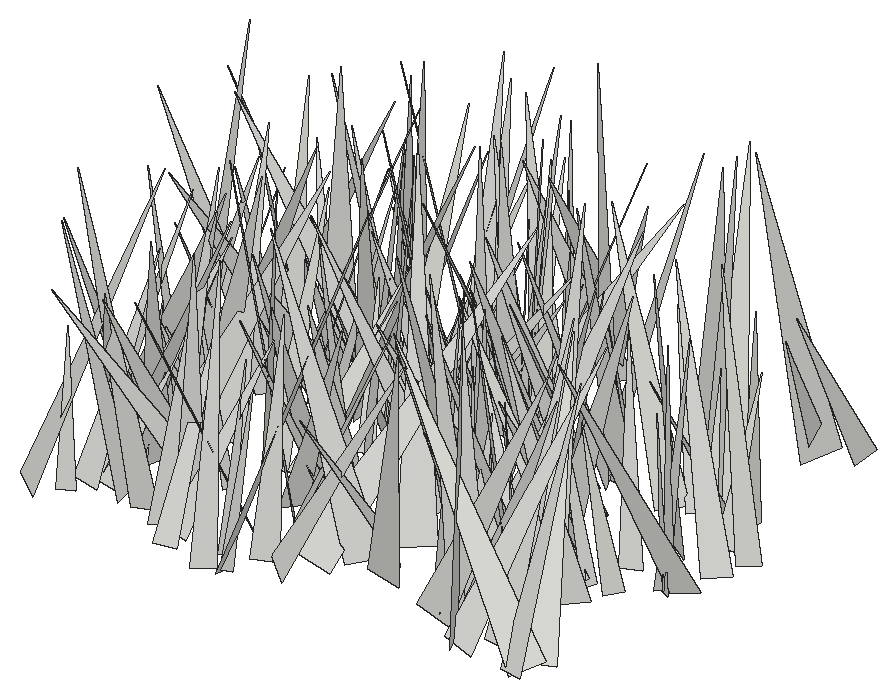
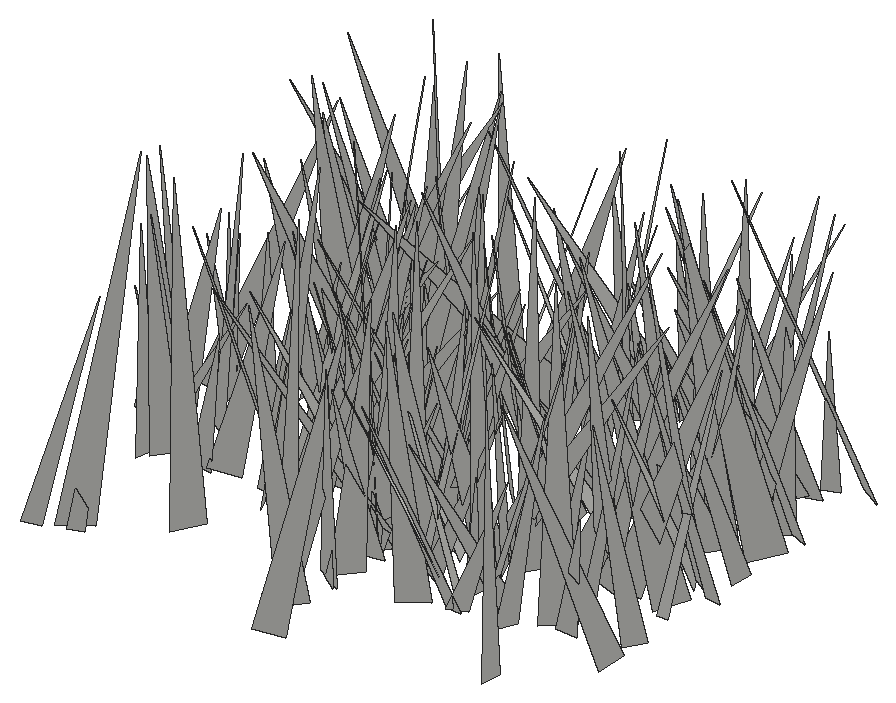
# SketchUp Ruby script. Lengths in inches.
U = 1.inch
M = Sketchup.active_model
def pt(a) = Geom::Point3d.new(a.map { |v| v * U })
def face(e, loops, mat)
  f = e.add_face(loops[0].map { |a| pt(a) })
  loops[1..].each { |l| e.add_face(l.map { |a| pt(a) }).erase! }
  f.material = f.back_material = mat if mat
  f
end
# faces: each face lists its corners as indices into pts; further lists are holes
def faces(e, pts, list, mat = nil) = list.each { |f| face(e, (f[0].is_a?(Array) ? f : [f]).map { |l| l.map { |i| pts[i] } }, mat) }
# xy, xz, yz: faces in a plane at the given z, y or x. An outline is a flat list of corners, or four numbers for a rectangle; further outlines are holes
def ring(l) = l.size == 4 ? [[l[0], l[1]], [l[2], l[1]], [l[2], l[3]], [l[0], l[3]]] : l.each_slice(2).to_a
def flat(e, list, mat, &to3) = list.each { |f| face(e, (f[0].is_a?(Array) ? f : [f]).map { |l| ring(l).map { |u, v| to3.(u, v) } }, mat) }
def xy(e, z, list, mat = nil) = flat(e, list, mat) { |x, y| [x, y, z] }
def xz(e, y, list, mat = nil) = flat(e, list, mat) { |x, z| [x, y, z] }
def yz(e, x, list, mat = nil) = flat(e, list, mat) { |y, z| [x, y, z] }
def lines(e, pts, list) = list.each { |a, b| e.add_line(pt(pts[a]), pt(pts[b])) }
# prism: a flat outline (further loops are holes) pulled along v
def prism(e, loops, v, mat = nil)
  f = face(e, loops, mat); d = Geom::Vector3d.new(v.map { |x| x * U })
  f.pushpull(f.normal.samedirection?(d) ? d.length : -d.length)
end
def box(e, o, s, mat = nil) = prism(e, [[o, [o[0] + s[0], o[1], o[2]], [o[0] + s[0], o[1] + s[1], o[2]], [o[0], o[1] + s[1], o[2]]]], [0, 0, s[2]], mat)
def at(x, y, z, deg = 0) = Geom::Transformation.translation(pt([x, y, z])) * Geom::Transformation.rotation(ORIGIN, Z_AXIS, deg.degrees)
def axes(o, x, y, z) = Geom::Transformation.new([*x, 0, *y, 0, *z, 0, *pt(o).to_a, 1])
def part(name) = M.definitions.add(name)
# library, detail: a bought-in or finely detailed component or shape, given as its bounding box
def library(name, o, s) = part(name).tap { |d| box(d.entities, o, s) }
def detail(e, o, s) = box(e.add_group.entities, o, s)
def put(e, d, t, mat = nil) = e.add_instance(d, t).tap { |i| i.material = mat if mat }
def group(e, t, mat = nil) = e.add_group.tap { |g| g.transformation = t; g.material = mat if mat }.entities
root = M.entities
c1 = part("fur_instance\#9")
p = [[0.8125,0,1.79],[0.67,-0.02,1.48],[0,-0.11,0],[0,0.11,0]]
faces(c1.entities,p,[[0,1,2,3]])
put(root,c1,axes([86.75,304.64,-27.1],[-1.48065,3.15767,1.46809],[3.42197,1.61497,-0.02236],[0.64523,-1.31889,3.48751]))
put(root,c1,axes([94.63,306.8,-27.1],[-3.64802,-5.0358,0.07825],[-5.03596,3.64854,0.02575],[0.06676,0.04827,6.21825]))
put(root,c1,axes([101.23,306.93,-27.1],[0.69431,-7.1025,1.01226],[-6.95299,-0.41552,1.85354],[1.7681,1.15502,6.89145]))
put(root,c1,axes([110.4,304.75,-27.1],[-5.51381,4.9525,0.02994],[4.6746,5.18943,2.47955],[-1.63592,-1.86355,6.98435]))
put(root,c1,axes([91.37,308.08,-27.1],[-6.30471,-1.37126,0.42808],[-1.05468,5.72683,2.8114],[0.97532,-2.67133,5.80738]))
put(root,c1,axes([88.87,305.9375,-27.1],[-6.26748,-0.84521,1.62615],[-0.68504,6.45447,0.7145],[1.69984,-0.51518,6.28372]))
put(root,c1,axes([106.66,304.7,-27.1],[6.19858,3.66698,3.16063],[3.75526,-6.8827,0.6206],[-3.05522,-1.01998,7.17523]))
put(root,c1,axes([95.93,303.48,-27.1],[-3.80527,0.70423,0.62745],[0.3357,3.44844,-1.83447],[0.88144,1.72686,3.40746]))
put(root,c1,axes([97.41,304.875,-27.1],[3.70489,5.29932,0.63458],[5.07029,-3.25343,-2.43293],[1.66665,-1.88258,5.99082]))
put(root,c1,axes([95.1,303.0625,-27.1],[-5.93651,2.05948,0.4431],[1.83167,5.70073,-1.95618],[1.04056,1.71471,5.97135]))
put(root,c1,axes([96.62,305.09,-27.1],[-2.20726,4.7722,2.01563],[5.04733,2.47451,-0.33147],[1.16667,-1.67676,5.24748]))
put(root,c1,axes([100.51,308.8,-27.1],[-3.99829,-3.957,0.07334],[-3.50173,3.58563,2.55553],[1.84422,-1.77059,5.01133]))
put(root,c1,axes([90.21,305.41,-27.1],[-1.59145,-6.67923,2.98055],[-7.18236,0.85085,-1.92829],[-1.38185,3.26993,6.58988]))
put(root,c1,axes([85.25,304,-27.1],[4.54632,6.46757,0.61256],[6.48609,-4.47646,-0.87508],[0.36794,-1.0028,7.85702]))
put(root,c1,axes([104.68,305.83,-27.1],[2.05152,-6.6713,2.37008],[-6.64568,-0.96384,3.03943],[2.44098,2.98279,6.28306]))
put(root,c1,axes([95.06,304.51,-27.1],[-3.85021,0.78609,0.9669],[0.45373,3.80886,-1.28983],[1.16059,1.11875,3.71193]))
put(root,c1,axes([92.46,304.58,-27.1],[0.05703,4.78722,0.58826],[4.57544,0.13244,-1.52137],[1.52606,-0.57598,4.5394]))
put(root,c1,axes([91.9375,306.15,-27.1],[5.0258,-2.8928,2.35137],[-3.11716,-5.42578,-0.01254],[-2.04464,1.16127,5.79886]))
put(root,c1,axes([92.71,303.54,-27.1],[-4.05374,2.9207,0.15477],[2.65047,3.78022,-1.91631],[1.23673,1.47198,4.61422]))
put(root,c1,axes([108.58,306.6875,-27.1],[-4.58076,1.47717,0.18742],[1.47131,4.39705,1.30451],[-0.22897,-1.29786,4.63288]))
put(root,c1,axes([110.08,304.04,-27.1],[1.80185,5.93958,0.37976],[5.89361,-1.83593,0.75111],[-0.82954,-0.14229,6.16126]))
put(root,c1,axes([89.45,309.17,-27.1],[5.03177,-2.92165,1.14225],[-2.20313,-4.82824,-2.64459],[-2.23316,-1.81978,5.18275]))
put(root,c1,axes([86.01,308.63,-27.1],[5.48383,-1.63022,0.30334],[-1.45467,-5.23263,-1.82362],[-0.79597,-1.66854,5.42259]))
put(root,c1,axes([88.15,308.71,-27.1],[6.15158,-3.29467,0.71793],[-3.15743,-6.15236,-1.17953],[-1.18361,-0.7112,6.87789]))
put(root,c1,axes([87,305.6,-27.1],[0.12132,5.40428,1.16344],[5.42728,0.10479,-1.05269],[1.05091,-1.16504,5.30215]))
put(root,c1,axes([105.55,306.79,-27.1],[-7.11208,1.53537,2.26223],[1.65379,7.4363,0.15223],[2.17716,-0.6331,7.27433]))
put(root,c1,axes([105.69,307.03,-27.1],[3.10657,-5.20372,2.6425],[-5.63717,-3.45056,-0.16782],[-1.51121,2.17421,6.05816]))
put(root,c1,axes([107.08,304.44,-27.1],[1.06363,7.1406,0.14161],[6.98782,-1.01087,-1.51263],[1.47601,-0.35985,7.05914]))
put(root,c1,axes([105.9,306.92,-27.1],[5.04993,-3.13211,0.88061],[-3.25342,-4.87587,1.31476],[-0.02926,1.58216,5.79512]))
put(root,c1,axes([95.79,303.2,-27.1],[6.81061,4.1437,0.72104],[3.52808,-6.3754,3.31382],[-2.28972,2.50169,7.25074]))
put(root,c1,axes([91.59,304.95,-27.1],[-6.63675,3.07759,1.929],[2.57186,6.8191,-2.03087],[2.56478,1.12578,7.02806]))
put(root,c1,axes([108.1,306.99,-27.1],[-5.99226,-3.56649,1.99916],[-3.93709,5.99,-1.11487],[1.10264,2.00593,6.88361]))
put(root,c1,axes([99.76,307.56,-27.1],[-4.16416,5.80884,2.0419],[6.1268,3.66414,2.07088],[-0.6118,-2.84317,6.84063]))
put(root,c1,axes([103.8,310.01,-27.1],[-0.44109,-6.89492,0.21564],[-6.89758,0.44393,0.08524],[0.09888,0.20974,6.90849]))
put(root,c1,axes([87.5,306.84,-27.1],[6.84085,-1.05323,0.60817],[-1.14548,-6.7472,1.19982],[-0.40871,1.28156,6.81667]))
put(root,c1,axes([108.29,305.54,-27.1],[1.00933,7.00307,0.82634],[7.04916,-1.02422,0.06983],[-0.18746,-0.80782,7.07509]))
put(root,c1,axes([87.49,306.01,-27.1],[-0.99691,5.86129,1.26655],[5.41282,1.43213,-2.36709],[2.58075,-0.73958,5.45394]))
put(root,c1,axes([105.18,307.28,-27.1],[2.53545,-3.02814,1.98338],[-3.53036,-2.60371,0.53779],[-0.80002,1.89288,3.91266]))
put(root,c1,axes([108.45,308.1,-27.1],[-2.5015,-6.23633,1.72664],[-6.18785,1.76379,-2.59425],[-1.89304,2.47545,6.19832]))
put(root,c1,axes([110.48,305.32,-27.1],[-3.69849,5.78351,0.10997],[5.76561,3.69627,-0.48502],[0.46777,0.16892,6.84781]))
put(root,c1,axes([87.125,309.52,-27.1],[-0.56263,-5.96411,0.83016],[-5.9756,0.45013,-0.816],[-0.74291,0.89616,5.93475]))
put(root,c1,axes([95.91,307.79,-27.1],[5.05169,2.87341,0.23488],[2.86098,-4.93803,-1.1233],[0.35552,-1.09113,5.70213]))
put(root,c1,axes([95.61,310.51,-27.1],[-4.40501,-3.46188,0.56585],[-3.18391,4.32713,1.68747],[1.47225,-1.00011,5.34239]))
put(root,c1,axes([104.59,306.125,-27.1],[3.23969,5.31398,1.47982],[4.81259,-3.56155,2.25346],[-2.69577,0.02794,5.80137]))
put(root,c1,axes([95.23,308.68,-27.1],[-5.96506,-5.04673,2.13711],[-5.35643,6.03696,-0.69462],[1.15994,1.92465,7.7826]))
put(root,c1,axes([87.87,308.01,-27.1],[1.06055,3.50039,1.15885],[3.68372,-1.05849,-0.17402],[-0.16095,-1.16074,3.65339]))
put(root,c1,axes([106.7,308.75,-27.1],[-3.07228,-3.20464,1.70758],[-3.41257,3.31254,0.07678],[1.24093,1.17551,4.43878]))
put(root,c1,axes([94.75,309.3,-27.1],[4.6953,-3.04636,0.27903],[-3.0591,-4.67738,0.40996],[-0.01004,0.49581,5.58194]))
put(root,c1,axes([103.18,309.26,-27.1],[-1.62958,-3.15436,1.09529],[-3.33909,1.53504,-0.54711],[-0.01197,1.22427,3.50802]))
put(root,c1,axes([92.86,309.88,-27.1],[6.58164,2.52237,2.667],[2.99732,-6.85363,-0.91486],[-2.11926,-1.85972,6.9888]))
put(root,c1,axes([108.49,310.15,-27.1],[-3.08305,4.83073,2.80211],[5.58378,2.72141,1.452],[0.09585,-3.15451,5.54372]))
put(root,c1,axes([107.08,308.8,-27.1],[-4.22119,3.06488,0.48562],[3.10212,4.18863,0.52921],[0.07866,-0.71394,5.1896]))
put(root,c1,axes([85.35,310.52,-27.1],[4.73655,-6.32836,0.37656],[-6.13582,-4.45802,2.25891],[1.59428,1.644,7.57499]))
put(root,c1,axes([87.41,310.73,-27.1],[0.83878,-6.84447,1.51714],[-6.71971,-0.34936,2.13903],[1.99848,1.69801,6.55552]))
put(root,c1,axes([85.33,308.53,-27.1],[3.14685,5.37097,0.90824],[5.43729,-3.03382,-0.89816],[0.32882,-1.23429,6.15981]))
put(root,c1,axes([88.83,311.11,-27.1],[2.63547,-2.52355,0.88422],[-2.24578,-2.7628,-1.19134],[-1.45143,-0.30736,3.44888]))
put(root,c1,axes([94.06,311.8,-27.1],[0.0355,-6.28923,0.69696],[-6.32457,-0.05728,-0.19472],[-0.19984,0.69551,6.28631]))
put(root,c1,axes([89.85,308.79,-27.1],[-6.30755,-1.0303,0.95825],[-1.23667,6.15876,-1.51833],[0.67114,1.66527,6.20817]))
put(root,c1,axes([91.82,308.8,-27.1],[-4.16837,-0.36819,0.02902],[-0.35612,3.91965,-1.4217],[-0.09791,1.41863,3.93569]))
put(root,c1,axes([101.26,312.25,-27.1],[-1.0754,-7.3325,1.08617],[-7.40599,1.10888,0.15329],[0.31086,1.05196,7.40935]))
put(root,c1,axes([95.22,312.34,-27.1],[3.85472,-3.45884,0.89823],[-3.26491,-3.94586,-1.18314],[-1.45282,-0.30973,5.04209]))
put(root,c1,axes([98.12,306.18,-27.1],[-4.06981,7.2471,0.38585],[5.9474,3.58401,-4.58433],[4.15906,1.9665,6.9331]))
put(root,c1,axes([111.46,313.57,-27.1],[1.05272,-6.58483,0.46236],[-6.33643,-1.13928,-1.79827],[-1.85027,0.15508,6.42141]))
put(root,c1,axes([109.25,311.74,-27.1],[2.35364,-2.97334,1.61897],[-3.0072,-2.74184,-0.66374],[-1.55518,0.80187,3.73361]))
put(root,c1,axes([105.82,313.24,-27.1],[1.37303,-5.10418,0.31363],[-5.09334,-1.39399,-0.38851],[-0.45708,0.20095,5.27134]))
put(root,c1,axes([102.78,310.7,-27.1],[1.15906,3.62365,1.13013],[3.60388,-1.42153,0.86183],[-1.19166,-0.77453,3.7056]))
put(root,c1,axes([106.47,310.68,-27.1],[5.95771,-4.00613,4.25574],[-5.13988,-6.48421,1.09155],[-2.78246,3.40011,7.09591]))
put(root,c1,axes([87.35,313.3125,-27.1],[2.07111,-6.85146,1.31632],[-6.80663,-1.68294,1.94991],[1.53132,1.78604,6.88693]))
put(root,c1,axes([108.1,311.6,-27.1],[-4.0966,0.35691,0.30901],[0.31396,4.07547,-0.54495],[0.35257,0.51784,4.07585]))
put(root,c1,axes([103.57,313.69,-27.1],[-0.91918,-4.72146,0.08029],[-4.18667,0.777,-2.23865],[-2.18412,0.49761,4.25741]))
put(root,c1,axes([96.03,311.35,-27.1],[-5.27526,-0.92635,0.94955],[-1.13263,5.17215,-1.24665],[0.69057,1.40673,5.20887]))
put(root,c1,axes([104.77,314.49,-27.1],[2.5877,-3.76016,0.15432],[-3.53923,-2.49522,-1.45139],[-1.27925,-0.70276,4.32764]))
put(root,c1,axes([100.7,309.81,-27.1],[-7.32021,3.8589,0.48336],[3.73123,7.2592,-1.44642],[1.09666,1.05977,8.14767]))
put(root,c1,axes([107.57,311.35,-27.1],[-2.18408,5.95276,0.46734],[5.01759,1.55993,3.57972],[-3.2369,-1.59851,5.23366]))
put(root,c1,axes([87.36,311.43,-27.1],[0.42432,7.03314,2.02201],[6.63788,0.48281,-3.07232],[3.08094,-2.00885,6.34082]))
put(root,c1,axes([85,312.58,-27.1],[4.99939,-0.31235,0.02616],[-0.31267,-4.999,0.06629],[-0.02197,0.06779,5.0087]))
put(root,c1,axes([92.18,311.3,-27.1],[0.04484,6.03011,0.93276],[6.10111,-0.02998,-0.09948],[0.09373,-0.93336,6.02946]))
put(root,c1,axes([99.77,313.04,-27.1],[-2.20634,6.02099,1.75888],[5.48729,0.94934,3.63349],[-3.03901,-2.65713,5.28374]))
put(root,c1,axes([98.72,315.29,-27.1],[3.46257,-3.0651,1.27719],[-2.41097,-3.5895,-2.07802],[-2.28326,-0.85797,4.13111]))
put(root,c1,axes([89.42,311.83,-27.1],[-0.62472,6.74476,1.37593],[6.88336,0.62526,0.06028],[0.06565,-1.37569,6.77336]))
put(root,c1,axes([93.52,311.24,-27.1],[-0.37436,5.47936,0.25355],[5.20879,0.43477,-1.70506],[1.71934,-0.12411,5.22075]))
put(root,c1,axes([110.82,313.04,-27.1],[1.66971,3.21733,1.57549],[3.35444,-2.01427,0.55833],[-1.25742,-1.10127,3.58153]))
put(root,c1,axes([98.45,312.81,-27.1],[1.87849,6.8023,2.53671],[7.02619,-2.36292,1.13321],[-1.82724,-2.09291,6.96533]))
put(root,c1,axes([102.99,313.41,-27.1],[-3.64875,-2.02244,1.121],[-2.25149,3.58457,-0.86132],[0.52696,1.3118,4.08188]))
put(root,c1,axes([89.71,317.73,-27.1],[4.2838,-6.03866,0.74714],[-5.20831,-4.11147,-3.36808],[-3.14598,-1.41597,6.59337]))
put(root,c1,axes([98.96,313.27,-27.1],[-4.99068,-1.45127,1.21381],[-1.71677,4.91279,-1.18474],[0.79513,1.49823,5.06058]))
put(root,c1,axes([99.82,315.05,-27.1],[-0.19463,-4.95849,1.24268],[-5.00803,0.4343,0.94858],[1.02496,1.18047,4.8708]))
put(root,c1,axes([96.39,313.1,-27.1],[4.10758,4.73433,2.04961],[4.7509,-4.49256,0.85604],[-2.01089,-0.9434,6.20913]))
put(root,c1,axes([102.83,314.64,-27.1],[6.50661,-0.43072,0.76621],[-0.39332,-6.54513,-0.33931],[-0.78607,-0.29036,6.51202]))
put(root,c1,axes([104.26,317.13,-27.1],[-2.87377,-5.9267,0.11201],[-5.79461,2.83495,1.33509],[1.24935,-0.48389,6.44995]))
put(root,c1,axes([103.26,312.14,-27.1],[-3.36255,6.42423,2.20976],[5.77924,4.00105,-2.8377],[3.57129,-0.42595,6.67271]))
put(root,c1,axes([104.48,314.44,-27.1],[4.99795,-3.82327,1.26682],[-4.01963,-4.86241,1.18375],[-0.25457,1.71502,6.18026]))
put(root,c1,axes([110.68,313.48,-27.1],[-4.80095,-0.85986,1.55653],[-1.24807,4.82151,-1.18603],[1.26668,1.49164,4.73094]))
put(root,c1,axes([102.17,316.67,-27.1],[1.78326,-6.33726,0.7797],[-6.26284,-1.89367,-1.06754],[-1.24322,0.44943,6.49625]))
put(root,c1,axes([85.58,316.96,-27.1],[-2.3415,-4.6423,0.1365],[-4.37976,2.25803,1.66471],[1.54509,-0.63449,4.92568]))
put(root,c1,axes([108.52,313.74,-27.1],[-0.93822,4.8343,1.08723],[4.93478,0.81164,0.64956],[-0.44769,-1.18472,4.88147]))
put(root,c1,axes([97.93,315.9,-27.1],[4.25123,5.18566,4.75994],[6.35301,-5.22113,0.01405],[-3.03108,-3.67013,6.70551]))
put(root,c1,axes([93.1,313.26,-27.1],[8.11647,0.24258,0.67526],[0.10402,-7.98511,1.61836],[-0.70993,1.60345,7.95719]))
put(root,c1,axes([84.85,314.61,-27.1],[2.54446,5.11145,1.43196],[5.2695,-2.24073,-1.36501],[0.64019,-1.87187,5.54418]))
put(root,c1,axes([110.55,313.16,-27.1],[-4.99347,0.21503,1.45697],[-0.36457,4.80955,-1.95935],[1.42691,1.98134,4.59803]))
put(root,c1,axes([99.07,315.56,-27.1],[-2.91756,2.69263,1.56889],[3.08399,2.80363,0.92331],[0.448,-1.76443,3.86133]))
put(root,c1,axes([88.27,316.11,-27.1],[1.0703,-6.74535,2.51722],[-6.58595,-1.94546,-2.41292],[-2.90886,1.9228,6.3893]))
put(root,c1,axes([102.05,316.36,-27.1],[-4.72142,-2.258,0.83052],[-2.14472,4.77905,0.80066],[1.09019,-0.37724,5.17198]))
put(root,c1,axes([94.5,314.21,-27.1],[4.33311,5.30156,2.10924],[5.44411,-4.63436,0.46433],[-1.70794,-1.32191,6.83131]))
put(root,c1,axes([85.88,315.95,-27.1],[6.5822,-3.48627,0.04021],[-3.46978,-6.5418,0.80411],[0.34104,0.72931,7.40492]))
put(root,c1,axes([92.13,317.36,-27.1],[7.49694,-1.26912,1.50095],[-0.87324,-7.45265,-1.93987],[-1.76095,-1.70734,7.35199]))
put(root,c1,axes([104.23,314.63,-27.1],[4.8135,2.02359,1.54657],[1.94555,-5.05552,0.55956],[-1.64367,-0.05793,5.19149]))
put(root,c1,axes([98.9,315.92,-27.1],[-0.48959,-3.44443,1.08487],[-3.54488,0.6673,0.51889],[0.68909,0.98557,3.44014]))
put(root,c1,axes([103.34,316.3,-27.1],[-4.54236,-5.48641,0.31776],[-5.31376,4.27953,-2.06985],[-1.40202,1.55551,6.81539]))
put(root,c1,axes([86.07,313.93,-27.1],[3.67219,7.15908,2.03524],[7.27938,-3.92759,0.68132],[-1.55086,-1.48365,8.01705]))
put(root,c1,axes([94.33,314.5,-27.1],[-1.12302,3.48075,0.37457],[3.50037,1.10997,0.18007],[-0.0574,-0.41163,3.65299]))
put(root,c1,axes([86.4,313.78,-27.1],[4.4489,2.71988,0.66857],[2.4928,-4.41728,1.38241],[-1.27698,0.85286,5.02786]))
put(root,c1,axes([88.92,316.45,-27.1],[-1.01611,-5.1437,1.43202],[-5.3112,0.8243,-0.80778],[-0.54728,1.55038,5.1805]))
put(root,c1,axes([102.97,317.59,-27.1],[2.20766,-6.15742,1.48059],[-5.96151,-2.54967,-1.71445],[-2.13691,0.75174,6.31254]))
put(root,c1,axes([109.11,316.06,-27.1],[3.12486,4.78234,3.10342],[5.39282,-3.6275,0.15986],[-1.8492,-2.49745,5.71052]))
put(root,c1,axes([92.16,314.48,-27.1],[3.27247,4.57721,0.86039],[4.6176,-3.3258,0.13012],[-0.60735,-0.62316,5.62521]))
put(root,c1,axes([93.54,317.72,-27.1],[-7.87957,1.88276,1.17896],[2.17634,7.41366,2.70618],[0.44527,-2.91806,7.63603]))
put(root,c1,axes([96.59,317.16,-27.1],[-4.94323,1.53486,1.76986],[2.06825,4.80019,1.61379],[1.10026,-2.12747,4.91803]))
put(root,c1,axes([98.81,317.42,-27.1],[-3.02452,-1.82217,1.01563],[-1.34667,3.07159,1.50047],[1.5932,-0.86291,3.19635]))
put(root,c1,axes([96.05,315.39,-27.1],[4.06376,5.39951,0.02576],[4.83357,-3.62337,-3.0294],[2.40665,-1.8401,6.04083]))
put(root,c1,axes([95.84,318.23,-27.1],[4.75134,-2.11282,0.36953],[-1.90852,-4.57438,-1.61505],[-0.97883,-1.33672,4.94275]))
put(root,c1,axes([102.36,316.24,-27.1],[0.25275,3.74041,1.98428],[3.79537,-1.08135,1.55493],[-1.87703,-1.68284,3.41127]))
put(root,c1,axes([101.22,315.96,-27.1],[5.9616,4.7587,3.0284],[5.08757,-6.43918,0.10304],[-2.43578,-1.80245,7.62727]))
put(root,c1,axes([94.24,316.02,-27.1],[-5.6206,-6.05261,0.8091],[-5.56666,4.62654,-4.06048],[-2.5102,3.29256,7.1929]))
put(root,c1,axes([111.67,315.34,-27.1],[-1.94953,6.2532,0.70862],[6.08536,1.68405,1.8809],[-1.60411,-1.2111,6.27419]))
put(root,c1,axes([98.69,316.38,-27.1],[1.00735,6.64791,2.58508],[7.07427,-1.26504,0.49655],[-0.91221,-2.46923,6.70544]))
put(root,c1,axes([88.56,318,-27.1],[-3.05463,-4.97038,1.37571],[-5.09206,3.16016,0.11108],[0.81742,1.11209,5.83293]))
put(root,c1,axes([96.85,317.41,-27.1],[3.67258,4.04026,0.63824],[3.75616,-2.99162,-2.6759],[1.61937,-2.22383,4.75932]))
put(root,c1,axes([90,313.87,-27.1],[6.02604,4.35688,0.13616],[4.14402,-5.7981,2.12678],[-1.35204,1.64734,7.12547]))
put(root,c1,axes([103.22,318.99,-27.1],[-5.52274,-3.05851,1.02558],[-2.84433,5.57616,1.31266],[1.52186,-0.67738,6.17511]))
put(root,c1,axes([88.98,316.01,-27.1],[-0.28002,6.79198,1.74012],[7.00527,0.19856,0.35229],[-0.29175,-1.75129,6.78861]))
put(root,c1,axes([99.74,317.09,-27.1],[4.36053,2.62617,0.62372],[2.69593,-4.29581,-0.7602],[-0.13318,-0.97427,5.03319]))
put(root,c1,axes([89.6,316.79,-27.1],[5.1332,2.66859,0.80867],[2.72409,-5.16107,-0.26035],[-0.59552,-0.60587,5.77956]))
put(root,c1,axes([89.5,318.89,-27.1],[2.09335,-3.21544,0.11512],[-3.16402,-2.08217,-0.6229],[-0.58423,-0.24481,3.78592]))
put(root,c1,axes([104.1,318.88,-27.1],[-0.46017,-7.01963,1.64197],[-7.20868,0.46604,-0.02793],[0.07879,1.64032,7.03464]))
put(root,c1,axes([110.33,318.51,-27.1],[-1.30366,-3.70433,0.26528],[-3.50778,1.13584,-1.37745],[-1.21983,0.69265,3.67753]))
put(root,c1,axes([110.42,317.39,-27.1],[-0.72601,3.76819,0.7458],[3.80081,0.81458,-0.41575],[0.55615,-0.64789,3.8149]))
put(root,c1,axes([112.07,316.92,-27.1],[-0.60049,6.11637,0.8715],[5.86899,0.29123,2.00004],[-1.92986,-1.0175,5.81123]))
put(root,c1,axes([94.93,318.08,-27.1],[4.2362,2.18763,0.04516],[2.18011,-4.21144,-0.49393],[0.18673,-0.4595,4.74206]))
put(root,c1,axes([93.05,317.6,-27.1],[-5.05417,-1.27819,2.14403],[-1.86511,5.15169,-1.32541],[1.65892,1.89778,5.04199]))
put(root,c1,axes([97.76,319.55,-27.1],[6.10585,-2.9623,2.45846],[-2.96929,-6.55789,-0.52733],[-2.45002,0.56525,6.76598]))
put(root,c1,axes([106.72,318.6875,-27.1],[-3.37701,5.49526,1.43426],[5.6473,3.0721,1.52623],[-0.60248,-2.00587,6.26679]))
put(root,c1,axes([85.02,319.4,-27.1],[3.32524,-3.2763,0.88677],[-3.39381,-3.22791,0.80025],[-0.05063,1.1934,4.59902]))
put(root,c1,axes([98.41,319.13,-27.1],[-3.74017,-2.83655,2.38458],[-3.12746,4.23356,0.13062],[1.98777,1.32365,4.69232]))
put(root,c1,axes([98.09,319.76,-27.1],[-0.66847,-3.61729,0.84651],[-3.58891,0.40659,-1.09666],[-0.95975,0.99906,3.51127]))
put(root,c1,axes([88.46,320.06,-27.1],[5.05478,-5.09898,2.04992],[-5.28407,-5.27475,-0.09077],[-1.51011,1.38923,7.17929]))
put(root,c1,axes([110.14,319.39,-27.1],[-4.58199,0.67037,2.42399],[0.81188,5.16228,0.10702],[2.38033,-0.47034,4.62953]))
put(root,c1,axes([92.61,319.69,-27.1],[7.55648,0.00384,2.83421],[0.13477,-8.06186,-0.34839],[-2.831,-0.37353,7.54844]))
put(root,c1,axes([103.84,319.81,-27.1],[-3.08604,-1.58363,1.00431],[-1.62158,3.22493,0.10239],[0.94181,0.36349,3.46714]))
put(root,c1,axes([94.92,320.125,-27.1],[-1.35927,-4.19334,1.10265],[-4.18909,0.97193,-1.4678],[-1.11869,1.45561,4.1566]))
put(root,c1,axes([108.58,318.74,-27.1],[2.96295,7.07925,2.39249],[7.30087,-3.29107,0.69644],[-1.59283,-1.91622,7.64263]))
put(root,c1,axes([107.72,318.9375,-27.1],[-1.2405,4.10694,0.41743],[4.03089,1.11105,1.04764],[-0.89058,-0.69186,4.16031]))
put(root,c1,axes([92.15,319.73,-27.1],[-6.45817,-1.9042,0.82118],[-2.02073,6.38203,-1.093],[0.4658,1.28531,6.64374]))
put(root,c1,axes([100.18,318.23,-27.1],[-5.70534,2.42628,0.74712],[2.22137,5.6608,-1.42016],[1.22905,1.03174,6.03498]))
put(root,c1,axes([99.35,317.73,-27.1],[2.9038,6.51052,1.10748],[6.2299,-3.10193,1.9005],[-2.1913,-0.1914,6.87074]))
put(root,c1,axes([93.42,317.95,-27.1],[-5.22484,3.83291,1.4033],[3.4058,5.3502,-1.93269],[2.24967,0.80218,6.18505]))
put(root,c1,axes([98.45,319.42,-27.1],[-2.02202,5.92033,1.45384],[6.05855,1.78151,1.17164],[-0.67672,-1.74024,6.14542]))
put(root,c1,axes([94.71,321.27,-27.1],[-5.73221,-5.07274,1.73381],[-5.23258,5.8463,-0.19467],[1.1657,1.29813,7.652]))
put(root,c1,axes([98.41,320.29,-27.1],[2.1369,3.02619,1.55246],[3.28055,-2.31782,0.00255],[-0.89775,-1.26656,3.70461]))
put(root,c1,axes([109.38,318.6875,-27.1],[-5.51425,5.90533,1.65371],[5.90522,5.71303,-0.71018],[1.6541,-0.70927,8.04832]))
put(root,c1,axes([99.53,317.8125,-27.1],[5.91646,3.40669,0.5347],[3.12979,-5.75065,2.00759],[-1.44773,1.49011,6.52531]))
put(root,c1,axes([96.99,317.68,-27.1],[-7.37463,3.18086,0.67882],[2.84062,7.11825,-2.49505],[1.58417,2.04365,7.63399]))
put(root,c1,axes([93.55,319.13,-27.1],[0.65103,4.23875,0.31259],[3.78552,-0.72206,1.9071],[-1.9325,0.01355,3.84107]))
put(root,c1,axes([107.45,319.8,-27.1],[-5.34624,-2.21651,3.3319],[-3.00843,5.89263,-0.90721],[2.6389,2.22728,5.71596]))
put(root,c1,axes([97.42,319.25,-27.1],[2.23337,6.49328,0.05356],[5.9184,-2.0122,-2.84202],[2.67172,-0.9705,6.25089]))
put(root,c1,axes([102.76,319.2,-27.1],[4.44163,5.80553,0.93246],[5.82565,-4.50337,0.28854],[-0.79717,-0.56325,7.30404]))
put(root,c1,axes([92.73,321,-27.1],[4.81991,2.46867,0.79438],[2.57067,-4.76928,-0.77622],[-0.3421,-1.05666,5.35942]))
put(root,c1,axes([90.01,321.4375,-27.1],[-4.92159,1.07561,1.43405],[1.22896,5.07505,0.41117],[1.30503,-0.72281,5.02095]))
put(root,c1,axes([87.76,320.36,-27.1],[-1.23895,4.11427,0.01816],[3.97981,1.19363,1.09497],[-1.04341,-0.33255,4.15491]))
put(root,c1,axes([84.82,321.16,-27.1],[5.89255,-1.31891,0.46121],[-1.38894,-5.74659,1.31223],[-0.15186,1.38261,5.89404]))
put(root,c1,axes([91.5625,319.75,-27.1],[4.67368,1.9817,0.84614],[1.46066,-4.3994,2.23565],[-1.58416,1.79011,4.55767]))
put(root,c1,axes([92.39,321.61,-27.1],[-3.14834,2.92622,0.07201],[2.87738,3.07451,0.86494],[-0.53726,-0.68166,4.21031]))
put(root,c1,axes([105.02,323.08,-27.1],[6.65936,-3.07974,1.86174],[-3.09449,-6.89952,-0.34452],[-1.83712,0.458,7.32893]))
put(root,c1,axes([97.7,322.05,-27.1],[-5.4066,3.91291,1.98693],[4.14231,5.59139,0.26032],[1.44915,-1.38406,6.66892]))
put(root,c1,axes([97.77,320.38,-27.1],[-1.13883,5.42731,0.08742],[5.42427,1.13458,0.2244],[-0.2017,-0.13157,5.54096]))
put(root,c1,axes([100.52,322.375,-27.1],[-3.60643,-6.53276,3.39182],[-7.2869,3.70246,-0.61691],[1.0404,3.28673,7.43658]))
put(root,c1,axes([92.46,321.73,-27.1],[1.86244,4.7215,0.55373],[4.68693,-1.72429,-1.06173],[0.79484,-0.89561,4.96326]))
put(root,c1,axes([94.17,322.2,-27.1],[-2.76968,5.79414,2.34049],[6.07448,3.09716,-0.47899],[1.46654,-1.88589,6.4042]))
put(root,c1,axes([97.83,323.05,-27.1],[2.36348,3.65871,1.87372],[3.9267,-2.64879,0.21906],[-1.21573,-1.4425,4.3502]))
put(root,c1,axes([98.54,325.43,-27.1],[2.87814,-5.28951,1.31735],[-4.95416,-3.15966,-1.86304],[-2.27391,0.18887,5.72641]))
put(root,c1,axes([108.72,325.76,-27.1],[6.46231,-4.31648,2.52967],[-3.92803,-6.93665,-1.8017],[-3.09867,-0.20881,7.55958]))
put(root,c1,axes([97.8,325.39,-27.1],[2.89446,-5.47209,0.08006],[-5.31049,-2.7865,1.53693],[1.32243,0.78724,5.99662]))
put(root,c1,axes([93.53,320.68,-27.1],[4.16098,5.56887,0.17793],[5.30628,-4.02846,1.99315],[-1.69922,1.05685,6.65984]))
put(root,c1,axes([108.44,326.0625,-27.1],[4.1039,-1.37964,0.4984],[-1.03776,-3.77714,-1.91052],[-1.03675,-1.68037,3.88527]))
put(root,c1,axes([97.98,322.86,-27.1],[1.64216,5.46326,1.64146],[5.44457,-2.0108,1.24565],[-1.70244,-1.16093,5.56707]))
put(root,c1,axes([87.8,325.1875,-27.1],[5.74214,0.07937,1.80023],[0.34922,-5.94743,-0.85168],[-1.76782,-0.91707,5.67918]))
put(root,c1,axes([97.1,327.8125,-27.1],[5.11337,-4.37567,0.02712],[-4.08728,-4.79107,-2.37351],[-1.56248,-1.78687,6.29758]))
put(root,c1,axes([110.18,326.77,-27.1],[4.14247,-2.36814,0.94959],[-1.79033,-3.98803,-2.13546],[-1.81783,-1.46881,4.26707]))
